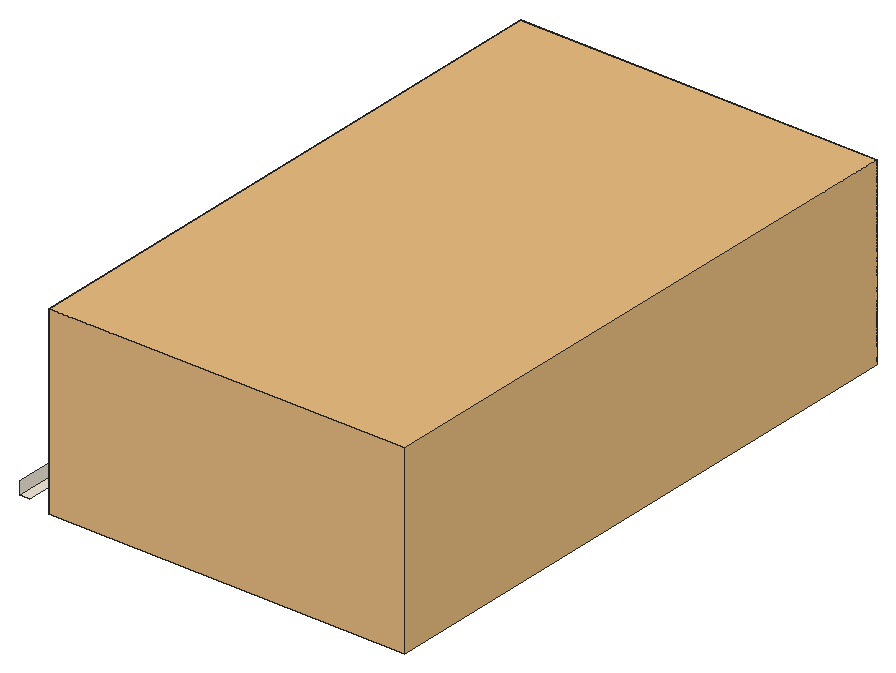
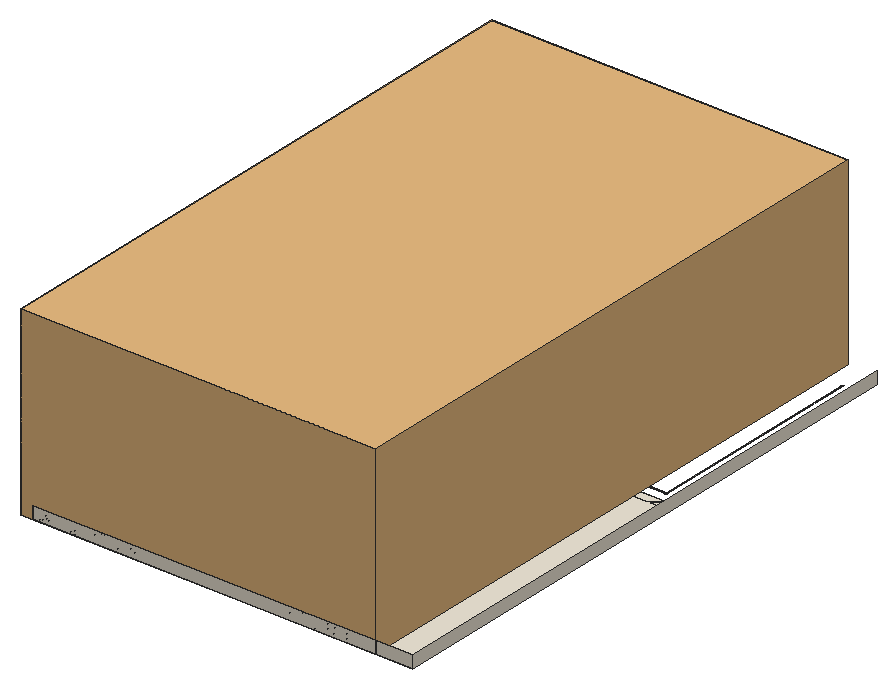
# SketchUp Ruby script. Lengths in inches.
U = 1.inch
M = Sketchup.active_model
def pt(a) = Geom::Point3d.new(a.map { |v| v * U })
def face(e, loops, mat)
  f = e.add_face(loops[0].map { |a| pt(a) })
  loops[1..].each { |l| e.add_face(l.map { |a| pt(a) }).erase! }
  f.material = f.back_material = mat if mat
  f
end
# faces: each face lists its corners as indices into pts; further lists are holes
def faces(e, pts, list, mat = nil) = list.each { |f| face(e, (f[0].is_a?(Array) ? f : [f]).map { |l| l.map { |i| pts[i] } }, mat) }
# xy, xz, yz: faces in a plane at the given z, y or x. An outline is a flat list of corners, or four numbers for a rectangle; further outlines are holes
def ring(l) = l.size == 4 ? [[l[0], l[1]], [l[2], l[1]], [l[2], l[3]], [l[0], l[3]]] : l.each_slice(2).to_a
def flat(e, list, mat, &to3) = list.each { |f| face(e, (f[0].is_a?(Array) ? f : [f]).map { |l| ring(l).map { |u, v| to3.(u, v) } }, mat) }
def xy(e, z, list, mat = nil) = flat(e, list, mat) { |x, y| [x, y, z] }
def xz(e, y, list, mat = nil) = flat(e, list, mat) { |x, z| [x, y, z] }
def yz(e, x, list, mat = nil) = flat(e, list, mat) { |y, z| [x, y, z] }
def lines(e, pts, list) = list.each { |a, b| e.add_line(pt(pts[a]), pt(pts[b])) }
# prism: a flat outline (further loops are holes) pulled along v
def prism(e, loops, v, mat = nil)
  f = face(e, loops, mat); d = Geom::Vector3d.new(v.map { |x| x * U })
  f.pushpull(f.normal.samedirection?(d) ? d.length : -d.length)
end
def box(e, o, s, mat = nil) = prism(e, [[o, [o[0] + s[0], o[1], o[2]], [o[0] + s[0], o[1] + s[1], o[2]], [o[0], o[1] + s[1], o[2]]]], [0, 0, s[2]], mat)
def at(x, y, z, deg = 0) = Geom::Transformation.translation(pt([x, y, z])) * Geom::Transformation.rotation(ORIGIN, Z_AXIS, deg.degrees)
def axes(o, x, y, z) = Geom::Transformation.new([*x, 0, *y, 0, *z, 0, *pt(o).to_a, 1])
def part(name) = M.definitions.add(name)
# library, detail: a bought-in or finely detailed component or shape, given as its bounding box
def library(name, o, s) = part(name).tap { |d| box(d.entities, o, s) }
def detail(e, o, s) = box(e.add_group.entities, o, s)
def put(e, d, t, mat = nil) = e.add_instance(d, t).tap { |i| i.material = mat if mat }
def group(e, t, mat = nil) = e.add_group.tap { |g| g.transformation = t; g.material = mat if mat }.entities
root = M.entities
M.materials.add("0027 AP L140 CRUSHED ICE").color = [241, 233, 217]
c1 = library("Group\#23",[36,0,-12],[348,576,180])
xy(root,120,[[9,214,18,456.5],[[9,214,18,214,18,456.5,88,456.5,88,456,99,456,99,456.5,100,456.5,100,456,165,456,165,300,381,300,381,780,9,780],[177,309,177,465,18,465,18,771,372,771,372,309]],[165,300,165,456,18,456,18,456.5,9,456.5,9,780,381,780,381,300]],"0027 AP L140 CRUSHED ICE")
xz(root,339,[[59.84,120,59.92,123],[59.92,120,60,123],[60,120,60.08,123],[60.08,120,60.16,123]],"0027 AP L140 CRUSHED ICE")
xz(root,411,[[59.84,120,59.92,123],[59.92,120,60,123],[60,120,60.08,123],[60.08,120,60.16,123]],"0027 AP L140 CRUSHED ICE")
xz(root,446,[[28,120,155,120.5]],"0027 AP L140 CRUSHED ICE")
xz(root,447,[[27,120,156,120.5]],"0027 AP L140 CRUSHED ICE")
xz(root,780,[[9,120,381,132]],"0027 AP L140 CRUSHED ICE")
yz(root,9,[[214,120,780,132]],"0027 AP L140 CRUSHED ICE")
yz(root,27,[[231,120,447,120.5]],"0027 AP L140 CRUSHED ICE")
yz(root,28,[[232,120,446,120.5]],"0027 AP L140 CRUSHED ICE")
yz(root,57,[[335.84,120,335.92,123],[335.92,120,336,123],[336,120,336.08,123],[336.08,120,336.16,123],[413.84,120,413.92,123],
  [413.92,120,414,123],[414,120,414.08,123],[414.08,120,414.16,123]],"0027 AP L140 CRUSHED ICE")
yz(root,63,[[335.84,120,335.92,123],[335.92,120,336,123],[336,120,336.08,123],[336.08,120,336.16,123],[413.84,120,413.92,123],
  [413.92,120,414,123]],"0027 AP L140 CRUSHED ICE")
yz(root,155,[[290,120,446,120.5]],"0027 AP L140 CRUSHED ICE")
yz(root,156,[[291,120,447,120.5]],"0027 AP L140 CRUSHED ICE")
yz(root,381,[[252,120,780,132]],"0027 AP L140 CRUSHED ICE")
p = [[57.36,334.57,120],[57.33,334.64,120],[57.33,334.64,123],[57.36,334.57,123],[57.29,334.71,120],[57.29,334.71,123],
  [62.67,334.64,120],[62.64,334.57,120],[62.64,334.57,123],[62.67,334.64,123],[62.71,334.71,120],[62.71,334.71,123],
  [57.26,334.78,120],[57.26,334.78,123],[62.74,334.78,120],[62.74,334.78,123],[57.23,334.85,120],[57.23,334.85,123],
  [62.77,334.85,120],[62.77,334.85,123],[57.2,334.92,120],[57.2,334.92,123],[57.17,335,120],[57.17,335,123],
  [62.8,334.92,120],[62.8,334.92,123],[62.83,335,120],[62.83,335,123],[57.15,335.07,120],[57.15,335.07,123],
  [62.85,335.07,120],[62.85,335.07,123],[57.125,335.15,120],[57.125,335.15,123],[57.1,335.22,120],[57.1,335.22,123],
  [62.875,335.15,120],[62.875,335.15,123],[62.9,335.22,120],[62.9,335.22,123],[57.08,335.3,120],[57.08,335.3,123],
  [62.92,335.3,120],[62.92,335.3,123],[57.07,335.375,120],[57.07,335.375,123],[62.93,335.375,120],[62.93,335.375,123],
  [57.05,335.45,120],[57.05,335.45,123],[62.95,335.45,120],[62.95,335.45,123],[57.04,335.53,120],[57.04,335.53,123],
  [57.03,335.61,120],[57.03,335.61,123],[62.96,335.53,120],[62.96,335.53,123],[62.97,335.61,120],[62.97,335.61,123],
  [57.02,335.6875,120],[57.02,335.6875,123],[62.98,335.6875,120],[62.98,335.6875,123],[57.01,335.76,120],[57.01,335.76,123],
  [62.99,335.76,120],[62.99,335.76,123],[57,335.84,120],[57,335.84,123],[63,335.84,120],[63,335.84,123],
  [57,336.16,120],[57.01,336.24,120],[57.01,336.24,123],[57,336.16,123],[57.02,336.3125,120],[57.02,336.3125,123],
  [62.99,336.24,120],[63,336.16,120],[63,336.16,123],[62.99,336.24,123],[62.98,336.3125,120],[62.98,336.3125,123],
  [57.03,336.39,120],[57.03,336.39,123],[62.97,336.39,120],[62.97,336.39,123],[57.04,336.47,120],[57.04,336.47,123],
  [62.96,336.47,120],[62.96,336.47,123],[57.05,336.55,120],[57.05,336.55,123],[57.07,336.625,120],[57.07,336.625,123],
  [62.95,336.55,120],[62.95,336.55,123],[62.93,336.625,120],[62.93,336.625,123],[57.08,336.7,120],[57.08,336.7,123],
  [62.92,336.7,120],[62.92,336.7,123],[57.1,336.78,120],[57.1,336.78,123],[62.9,336.78,120],[62.9,336.78,123],
  [57.125,336.85,120],[57.125,336.85,123],[62.875,336.85,120],[62.875,336.85,123],[57.15,336.93,120],[57.15,336.93,123],
  [57.17,337,120],[57.17,337,123],[62.83,337,120],[62.85,336.93,120],[62.85,336.93,123],[62.83,337,123],
  [57.2,337.08,120],[57.2,337.08,123],[62.8,337.08,120],[62.8,337.08,123],[57.23,337.15,120],[57.23,337.15,123],
  [57.26,337.22,120],[57.26,337.22,123],[62.74,337.22,120],[62.77,337.15,120],[62.77,337.15,123],[62.74,337.22,123],
  [57.29,337.29,120],[57.29,337.29,123],[62.71,337.29,120],[62.71,337.29,123],[57.33,337.36,120],[57.33,337.36,123],
  [62.67,337.36,120],[62.67,337.36,123],[57.36,337.43,120],[57.36,337.43,123],[57.4,337.5,120],[57.4,337.5,123],
  [62.64,337.43,120],[62.64,337.43,123],[62.6,337.5,120],[62.6,337.5,123],[57.44,337.57,120],[57.44,337.57,123],
  [62.56,337.57,120],[62.56,337.57,123],[57.48,337.63,120],[57.48,337.63,123],[57.53,337.7,120],[57.53,337.7,123],
  [62.52,337.63,120],[62.52,337.63,123],[62.47,337.7,120],[62.47,337.7,123],[57.57,337.76,120],[57.57,337.76,123],
  [62.43,337.76,120],[62.43,337.76,123],[57.62,337.83,120],[57.62,337.83,123],[57.67,337.89,120],[57.67,337.89,123],
  [62.33,337.89,120],[62.38,337.83,120],[62.38,337.83,123],[62.33,337.89,123],[57.72,337.95,120],[57.72,337.95,123],
  [57.77,338.01,120],[57.77,338.01,123],[62.23,338.01,120],[62.28,337.95,120],[62.28,337.95,123],[62.23,338.01,123],
  [57.82,338.07,120],[57.82,338.07,123],[62.18,338.07,120],[62.18,338.07,123],[57.88,338.12,120],[57.88,338.12,123],
  [57.93,338.18,120],[57.93,338.18,123],[62.12,338.12,120],[62.12,338.12,123],[62.07,338.18,120],[62.07,338.18,123],
  [57.99,338.23,120],[57.99,338.23,123],[58.05,338.28,120],[58.05,338.28,123],[61.95,338.28,120],[62.01,338.23,120],
  [62.01,338.23,123],[61.95,338.28,123],[58.11,338.33,120],[58.11,338.33,123],[58.17,338.38,120],[58.17,338.38,123],
  [61.83,338.38,120],[61.89,338.33,120],[61.89,338.33,123],[61.83,338.38,123],[58.24,338.43,120],[58.24,338.43,123],
  [58.3,338.47,120],[58.3,338.47,123],[61.7,338.47,120],[61.76,338.43,120],[61.76,338.43,123],[61.7,338.47,123],
  [58.37,338.52,120],[58.37,338.52,123],[58.43,338.56,120],[58.43,338.56,123],[61.63,338.52,120],[61.63,338.52,123],
  [61.57,338.56,120],[61.57,338.56,123],[58.5,338.6,120],[58.5,338.6,123],[58.57,338.64,120],[58.57,338.64,123],
  [58.64,338.67,120],[58.64,338.67,123],[61.43,338.64,120],[61.5,338.6,120],[61.5,338.6,123],[61.43,338.64,123],
  [61.36,338.67,120],[61.36,338.67,123],[58.71,338.71,120],[58.71,338.71,123],[58.78,338.74,120],[58.78,338.74,123],
  [58.85,338.77,120],[58.85,338.77,123],[61.15,338.77,120],[61.22,338.74,120],[61.22,338.74,123],[61.15,338.77,123],
  [61.29,338.71,120],[61.29,338.71,123],[58.92,338.8,120],[58.92,338.8,123],[59,338.83,120],[59,338.83,123],
  [59.07,338.85,120],[59.07,338.85,123],[60.93,338.85,120],[61,338.83,120],[61,338.83,123],[60.93,338.85,123],
  [61.08,338.8,120],[61.08,338.8,123],[59.15,338.875,120],[59.15,338.875,123],[59.22,338.9,120],[59.22,338.9,123],
  [59.3,338.92,120],[59.3,338.92,123],[59.375,338.93,120],[59.375,338.93,123],[59.45,338.95,120],[59.45,338.95,123],
  [59.53,338.96,120],[59.53,338.96,123],[60.55,338.95,120],[60.625,338.93,120],[60.625,338.93,123],[60.55,338.95,123],
  [60.47,338.96,120],[60.47,338.96,123],[60.7,338.92,120],[60.7,338.92,123],[60.78,338.9,120],[60.78,338.9,123],
  [60.85,338.875,120],[60.85,338.875,123],[59.61,338.97,120],[59.61,338.97,123],[59.6875,338.98,120],[59.6875,338.98,123],
  [59.76,338.99,120],[59.76,338.99,123],[59.84,339,120],[59.84,339,123],[60.24,338.99,120],[60.3125,338.98,120],
  [60.3125,338.98,123],[60.24,338.99,123],[60.16,339,120],[60.16,339,123],[60.39,338.97,120],[60.39,338.97,123],
  [59.61,411.03,120],[59.53,411.04,120],[59.53,411.04,123],[59.61,411.03,123],[59.45,411.05,120],[59.45,411.05,123],
  [59.6875,411.02,120],[59.6875,411.02,123],[59.76,411.01,120],[59.76,411.01,123],[59.84,411,120],[59.84,411,123],
  [60.24,411.01,120],[60.16,411,120],[60.16,411,123],[60.24,411.01,123],[60.3125,411.02,120],[60.3125,411.02,123],
  [60.39,411.03,120],[60.39,411.03,123],[60.47,411.04,120],[60.47,411.04,123],[60.55,411.05,120],[60.55,411.05,123],
  [59.07,411.15,120],[59,411.17,120],[59,411.17,123],[59.07,411.15,123],[59.22,411.1,120],[59.15,411.125,120],
  [59.15,411.125,123],[59.22,411.1,123],[59.3,411.08,120],[59.3,411.08,123],[59.375,411.07,120],[59.375,411.07,123],
  [60.625,411.07,120],[60.625,411.07,123],[60.7,411.08,120],[60.7,411.08,123],[60.78,411.1,120],[60.78,411.1,123],
  [60.85,411.125,120],[60.85,411.125,123],[60.93,411.15,120],[60.93,411.15,123],[61,411.17,120],[61,411.17,123],
  [58.85,411.23,120],[58.78,411.26,120],[58.78,411.26,123],[58.85,411.23,123],[58.92,411.2,120],[58.92,411.2,123],
  [61.08,411.2,120],[61.08,411.2,123],[61.15,411.23,120],[61.15,411.23,123],[61.22,411.26,120],[61.22,411.26,123],
  [58.71,411.29,120],[58.64,411.33,120],[58.64,411.33,123],[58.71,411.29,123],[58.57,411.36,120],[58.57,411.36,123],
  [61.29,411.29,120],[61.29,411.29,123],[61.36,411.33,120],[61.36,411.33,123],[61.43,411.36,120],[61.43,411.36,123],
  [58.5,411.4,120],[58.43,411.44,120],[58.43,411.44,123],[58.5,411.4,123],[58.37,411.48,120],[58.37,411.48,123],
  [61.5,411.4,120],[61.5,411.4,123],[61.57,411.44,120],[61.57,411.44,123],[61.63,411.48,120],[61.63,411.48,123],
  [58.3,411.53,120],[58.24,411.57,120],[58.24,411.57,123],[58.3,411.53,123],[61.7,411.53,120],[61.7,411.53,123],
  [61.76,411.57,120],[61.76,411.57,123],[58.17,411.62,120],[58.11,411.67,120],[58.11,411.67,123],[58.17,411.62,123],
  [61.83,411.62,120],[61.83,411.62,123],[61.89,411.67,120],[61.89,411.67,123],[58.05,411.72,120],[57.99,411.77,120],
  [57.99,411.77,123],[58.05,411.72,123],[61.95,411.72,120],[61.95,411.72,123],[62.01,411.77,120],[62.01,411.77,123],
  [57.93,411.82,120],[57.93,411.82,123],[57.88,411.88,120],[57.88,411.88,123],[62.07,411.82,120],[62.07,411.82,123],
  [62.12,411.88,120],[62.12,411.88,123],[57.82,411.93,120],[57.82,411.93,123],[57.77,411.99,120],[57.77,411.99,123],
  [62.18,411.93,120],[62.18,411.93,123],[62.23,411.99,120],[62.23,411.99,123],[57.72,412.05,120],[57.72,412.05,123],
  [62.28,412.05,120],[62.28,412.05,123],[57.67,412.11,120],[57.62,412.17,120],[57.62,412.17,123],[57.67,412.11,123],
  [62.33,412.11,120],[62.33,412.11,123],[62.38,412.17,120],[62.38,412.17,123],[57.57,412.24,120],[57.53,412.3,120],
  [57.53,412.3,123],[57.57,412.24,123],[62.43,412.24,120],[62.43,412.24,123],[62.47,412.3,120],[62.47,412.3,123],
  [57.48,412.37,120],[57.48,412.37,123],[62.52,412.37,120],[62.52,412.37,123],[57.44,412.43,120],[57.44,412.43,123],
  [57.4,412.5,120],[57.4,412.5,123],[62.56,412.43,120],[62.56,412.43,123],[62.6,412.5,120],[62.6,412.5,123],
  [57.36,412.57,120],[57.36,412.57,123],[62.64,412.57,120],[62.64,412.57,123],[57.33,412.64,120],[57.33,412.64,123],
  [57.29,412.71,120],[57.29,412.71,123],[62.67,412.64,120],[62.67,412.64,123],[62.71,412.71,120],[62.71,412.71,123],
  [57.26,412.78,120],[57.26,412.78,123],[62.74,412.78,120],[62.74,412.78,123],[57.23,412.85,120],[57.23,412.85,123],
  [62.77,412.85,120],[62.77,412.85,123],[57.2,412.92,120],[57.2,412.92,123],[57.17,413,120],[57.17,413,123],
  [62.8,412.92,120],[62.8,412.92,123],[62.83,413,120],[62.83,413,123],[57.15,413.07,120],[57.15,413.07,123],
  [62.85,413.07,120],[62.85,413.07,123],[57.125,413.15,120],[57.125,413.15,123],[57.1,413.22,120],[57.1,413.22,123],
  [62.875,413.15,120],[62.875,413.15,123],[62.9,413.22,120],[62.9,413.22,123],[57.08,413.3,120],[57.08,413.3,123],
  [62.92,413.3,120],[62.92,413.3,123],[57.07,413.375,120],[57.07,413.375,123],[62.93,413.375,120],[62.93,413.375,123],
  [57.05,413.45,120],[57.05,413.45,123],[62.95,413.45,120],[62.95,413.45,123],[57.04,413.53,120],[57.04,413.53,123],
  [57.03,413.61,120],[57.03,413.61,123],[62.96,413.53,120],[62.96,413.53,123],[62.97,413.61,120],[62.97,413.61,123],
  [57.02,413.6875,120],[57.02,413.6875,123],[62.98,413.6875,120],[62.98,413.6875,123],[57.01,413.76,120],[57.01,413.76,123],
  [62.99,413.76,120],[62.99,413.76,123],[57,413.84,120],[57,413.84,123],[63,413.84,120],[63,413.84,123],
  [57,414.16,120],[57.01,414.24,120],[57.01,414.24,123],[57,414.16,123],[57.02,414.3125,120],[57.02,414.3125,123],
  [57.03,414.39,120],[57.03,414.39,123],[57.04,414.47,120],[57.04,414.47,123],[57.05,414.55,120],[57.05,414.55,123],
  [57.07,414.625,120],[57.07,414.625,123],[57.08,414.7,120],[57.08,414.7,123],[57.1,414.78,120],[57.1,414.78,123],
  [57.125,414.85,120],[57.125,414.85,123],[57.15,414.93,120],[57.15,414.93,123],[57.17,415,120],[57.17,415,123],
  [57.2,415.08,120],[57.2,415.08,123],[57.23,415.15,120],[57.23,415.15,123],[57.26,415.22,120],[57.26,415.22,123],
  [57.29,415.29,120],[57.29,415.29,123],[57.33,415.36,120],[57.33,415.36,123],[57.36,415.43,120],[57.36,415.43,123],
  [57.4,415.5,120],[57.4,415.5,123],[57.44,415.57,120],[57.44,415.57,123],[57.48,415.63,120],[57.48,415.63,123],
  [57.53,415.7,120],[57.53,415.7,123],[57.57,415.76,120],[57.57,415.76,123],[57.62,415.83,120],[57.62,415.83,123],
  [57.67,415.89,120],[57.67,415.89,123],[57.72,415.95,120],[57.72,415.95,123],[57.77,416.01,120],[57.77,416.01,123],
  [57.82,416.07,120],[57.82,416.07,123],[57.88,416.12,120],[57.88,416.12,123],[57.93,416.18,120],[57.93,416.18,123],
  [57.99,416.23,120],[57.99,416.23,123],[58.05,416.28,120],[58.05,416.28,123],[58.11,416.33,120],[58.11,416.33,123],
  [58.17,416.38,120],[58.17,416.38,123],[58.24,416.43,120],[58.24,416.43,123],[58.3,416.47,120],[58.3,416.47,123],
  [58.37,416.52,120],[58.37,416.52,123],[58.43,416.56,120],[58.43,416.56,123],[58.5,416.6,120],[58.5,416.6,123],
  [58.57,416.64,120],[58.57,416.64,123],[58.64,416.67,120],[58.64,416.67,123],[58.71,416.71,120],[58.71,416.71,123],
  [58.78,416.74,120],[58.78,416.74,123],[58.85,416.77,120],[58.85,416.77,123],[58.92,416.8,120],[58.92,416.8,123],
  [59,416.83,120],[59,416.83,123],[59.07,416.85,120],[59.07,416.85,123],[59.15,416.875,120],[59.15,416.875,123],
  [59.22,416.9,120],[59.22,416.9,123],[59.3,416.92,120],[59.3,416.92,123],[59.375,416.93,120],[59.375,416.93,123],
  [165,456.5,120],[165,456,120]]
faces(root,p,[[0,1,2,3],[1,4,5,2],[6,7,8,9],[10,6,9,11],[4,12,13,5],[14,10,11,15],[12,16,17,13],[18,14,15,19],
  [16,20,21,17],[20,22,23,21],[24,18,19,25],[26,24,25,27],[22,28,29,23],[30,26,27,31],[28,32,33,29],[32,34,35,33],
  [36,30,31,37],[38,36,37,39],[34,40,41,35],[42,38,39,43],[40,44,45,41],[46,42,43,47],[44,48,49,45],[50,46,47,51],
  [48,52,53,49],[52,54,55,53],[56,50,51,57],[58,56,57,59],[54,60,61,55],[62,58,59,63],[60,64,65,61],[66,62,63,67],
  [64,68,69,65],[70,66,67,71],[72,73,74,75],[73,76,77,74],[78,79,80,81],[82,78,81,83],[76,84,85,77],[86,82,83,87],
  [84,88,89,85],[90,86,87,91],[88,92,93,89],[92,94,95,93],[96,90,91,97],[98,96,97,99],[94,100,101,95],[102,98,99,103],
  [100,104,105,101],[106,102,103,107],[104,108,109,105],[110,106,107,111],[108,112,113,109],[112,114,115,113],[116,117,118,119],[117,110,111,118],
  [114,120,121,115],[122,116,119,123],[120,124,125,121],[124,126,127,125],[128,129,130,131],[129,122,123,130],[126,132,133,127],[134,128,131,135],
  [132,136,137,133],[138,134,135,139],[136,140,141,137],[140,142,143,141],[144,138,139,145],[146,144,145,147],[142,148,149,143],[150,146,147,151],
  [148,152,153,149],[152,154,155,153],[156,150,151,157],[158,156,157,159],[154,160,161,155],[162,158,159,163],[160,164,165,161],[164,166,167,165],
  [168,169,170,171],[169,162,163,170],[166,172,173,167],[172,174,175,173],[176,177,178,179],[177,168,171,178],[174,180,181,175],[182,176,179,183],
  [180,184,185,181],[184,186,187,185],[188,182,183,189],[190,188,189,191],[186,192,193,187],[192,194,195,193],[196,197,198,199],[197,190,191,198],
  [194,200,201,195],[200,202,203,201],[204,205,206,207],[205,196,199,206],[202,208,209,203],[208,210,211,209],[212,213,214,215],[213,204,207,214],
  [210,216,217,211],[216,218,219,217],[220,212,215,221],[222,220,221,223],[218,224,225,219],[224,226,227,225],[226,228,229,227],[230,231,232,233],
  [234,230,233,235],[231,222,223,232],[228,236,237,229],[236,238,239,237],[238,240,241,239],[242,243,244,245],[243,246,247,244],[246,234,235,247],
  [240,248,249,241],[248,250,251,249],[250,252,253,251],[254,255,256,257],[255,258,259,256],[258,242,245,259],[252,260,261,253],[260,262,263,261],
  [262,264,265,263],[264,266,267,265],[266,268,269,267],[268,270,271,269],[272,273,274,275],[276,272,275,277],[273,278,279,274],[278,280,281,279],
  [280,282,283,281],[282,254,257,283],[270,284,285,271],[284,286,287,285],[286,288,289,287],[288,290,291,289],[292,293,294,295],[296,292,295,297],
  [293,298,299,294],[298,276,277,299],[300,301,302,303],[301,304,305,302],[306,300,303,307],[308,306,307,309],[310,308,309,311],[312,313,314,315],
  [316,312,315,317],[318,316,317,319],[320,318,319,321],[322,320,321,323],[324,325,326,327],[328,329,330,331],[329,324,327,330],[332,328,331,333],
  [334,332,333,335],[304,334,335,305],[336,322,323,337],[338,336,337,339],[340,338,339,341],[342,340,341,343],[344,342,343,345],[346,344,345,347],
  [348,349,350,351],[325,352,353,326],[352,348,351,353],[354,346,347,355],[356,354,355,357],[358,356,357,359],[360,361,362,363],[361,364,365,362],
  [349,360,363,350],[366,358,359,367],[368,366,367,369],[370,368,369,371],[372,373,374,375],[373,376,377,374],[364,372,375,365],[378,370,371,379],
  [380,378,379,381],[382,380,381,383],[384,385,386,387],[376,384,387,377],[388,382,383,389],[390,388,389,391],[392,393,394,395],[385,392,395,386],
  [396,390,391,397],[398,396,397,399],[400,401,402,403],[393,400,403,394],[404,398,399,405],[406,404,405,407],[401,408,409,402],[408,410,411,409],
  [412,406,407,413],[414,412,413,415],[410,416,417,411],[416,418,419,417],[420,414,415,421],[422,420,421,423],[418,424,425,419],[426,422,423,427],
  [428,429,430,431],[424,428,431,425],[432,426,427,433],[434,432,433,435],[436,437,438,439],[429,436,439,430],[440,434,435,441],[442,440,441,443],
  [437,444,445,438],[446,442,443,447],[444,448,449,445],[448,450,451,449],[452,446,447,453],[454,452,453,455],[450,456,457,451],[458,454,455,459],
  [456,460,461,457],[460,462,463,461],[464,458,459,465],[466,464,465,467],[462,468,469,463],[470,466,467,471],[468,472,473,469],[474,470,471,475],
  [472,476,477,473],[476,478,479,477],[480,474,475,481],[482,480,481,483],[478,484,485,479],[486,482,483,487],[484,488,489,485],[488,490,491,489],
  [492,486,487,493],[494,492,493,495],[490,496,497,491],[498,494,495,499],[496,500,501,497],[502,498,499,503],[500,504,505,501],[506,502,503,507],
  [504,508,509,505],[508,510,511,509],[512,506,507,513],[514,512,513,515],[510,516,517,511],[518,514,515,519],[516,520,521,517],[522,518,519,523],
  [520,524,525,521],[526,522,523,527],[528,529,530,531],[529,532,533,530],[532,534,535,533],[534,536,537,535],[536,538,539,537],[538,540,541,539],
  [540,542,543,541],[542,544,545,543],[544,546,547,545],[546,548,549,547],[548,550,551,549],[550,552,553,551],[552,554,555,553],[554,556,557,555],
  [556,558,559,557],[558,560,561,559],[560,562,563,561],[562,564,565,563],[564,566,567,565],[566,568,569,567],[568,570,571,569],[570,572,573,571],
  [572,574,575,573],[574,576,577,575],[576,578,579,577],[578,580,581,579],[580,582,583,581],[582,584,585,583],[584,586,587,585],[586,588,589,587],
  [588,590,591,589],[590,592,593,591],[592,594,595,593],[594,596,597,595],[596,598,599,597],[598,600,601,599],[600,602,603,601],[602,604,605,603],
  [604,606,607,605],[606,608,609,607],[608,610,611,609],[610,612,613,611],[612,614,615,613],[614,616,617,615],[616,618,619,617],[618,620,621,619],
  [620,622,623,621],[622,624,625,623],[624,626,627,625],[626,628,629,627]],"0027 AP L140 CRUSHED ICE")
lines(root,p,[[630,631]])
put(root,c1,at(9,204,132),"0027 AP L140 CRUSHED ICE")
